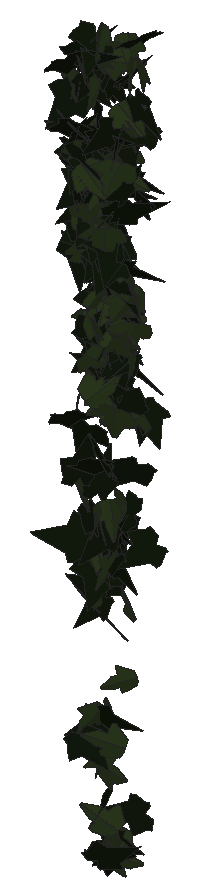
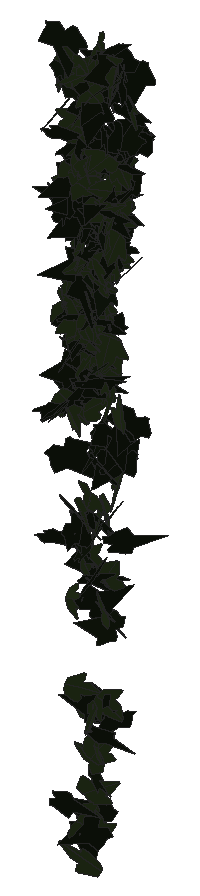
# SketchUp Ruby script. Lengths in millimetres.
U = 1.mm
M = Sketchup.active_model
def pt(a) = Geom::Point3d.new(a.map { |v| v * U })
def face(e, loops, mat)
  f = e.add_face(loops[0].map { |a| pt(a) })
  loops[1..].each { |l| e.add_face(l.map { |a| pt(a) }).erase! }
  f.material = f.back_material = mat if mat
  f
end
# faces: each face lists its corners as indices into pts; further lists are holes
def faces(e, pts, list, mat = nil) = list.each { |f| face(e, (f[0].is_a?(Array) ? f : [f]).map { |l| l.map { |i| pts[i] } }, mat) }
# xy, xz, yz: faces in a plane at the given z, y or x. An outline is a flat list of corners, or four numbers for a rectangle; further outlines are holes
def ring(l) = l.size == 4 ? [[l[0], l[1]], [l[2], l[1]], [l[2], l[3]], [l[0], l[3]]] : l.each_slice(2).to_a
def flat(e, list, mat, &to3) = list.each { |f| face(e, (f[0].is_a?(Array) ? f : [f]).map { |l| ring(l).map { |u, v| to3.(u, v) } }, mat) }
def xy(e, z, list, mat = nil) = flat(e, list, mat) { |x, y| [x, y, z] }
def xz(e, y, list, mat = nil) = flat(e, list, mat) { |x, z| [x, y, z] }
def yz(e, x, list, mat = nil) = flat(e, list, mat) { |y, z| [x, y, z] }
def lines(e, pts, list) = list.each { |a, b| e.add_line(pt(pts[a]), pt(pts[b])) }
# prism: a flat outline (further loops are holes) pulled along v
def prism(e, loops, v, mat = nil)
  f = face(e, loops, mat); d = Geom::Vector3d.new(v.map { |x| x * U })
  f.pushpull(f.normal.samedirection?(d) ? d.length : -d.length)
end
def box(e, o, s, mat = nil) = prism(e, [[o, [o[0] + s[0], o[1], o[2]], [o[0] + s[0], o[1] + s[1], o[2]], [o[0], o[1] + s[1], o[2]]]], [0, 0, s[2]], mat)
def at(x, y, z, deg = 0) = Geom::Transformation.translation(pt([x, y, z])) * Geom::Transformation.rotation(ORIGIN, Z_AXIS, deg.degrees)
def axes(o, x, y, z) = Geom::Transformation.new([*x, 0, *y, 0, *z, 0, *pt(o).to_a, 1])
def part(name) = M.definitions.add(name)
# library, detail: a bought-in or finely detailed component or shape, given as its bounding box
def library(name, o, s) = part(name).tap { |d| box(d.entities, o, s) }
def detail(e, o, s) = box(e.add_group.entities, o, s)
def put(e, d, t, mat = nil) = e.add_instance(d, t).tap { |i| i.material = mat if mat }
def group(e, t, mat = nil) = e.add_group.tap { |g| g.transformation = t; g.material = mat if mat }.entities
root = M.entities
M.materials.add("efeu1").color = [18, 25, 13]
M.materials.add("efeu2").color = [43, 57, 29]
c1 = part("ivyleaf_10")
p = [[0,12.8,-0.8],[-1.5,51.3,-10.9],[-4.9,51,-11.6],[-13.6,26.5,-7.3],[-13.2,15.9,-4.6],[-21.1,19.3,-7.2],
  [-29.5,16.3,-8.3],[-29.2,8.3,-6.2],[-19.7,-9.8,0.5],[-7.6,-13,4],[1,-12.2,5.8],[-0.4,51.1,-11.1],
  [-1.5,51.1,-10.9],[1,-12.4,5.9],[16.9,-12.4,3.5],[35.1,9.1,-5.1],[35,12.9,-6.1],[20.5,16.4,-4.9],
  [15.8,15,-3.8],[15.3,27.6,-7.1],[12.8,31.3,-7.8]]
faces(c1.entities,p,[[0,1,2,3,4,5,6,7,8,9,10],[11,12,0,13,14,15,16,17,18,19,20]],"efeu2")
c2 = part("ivyleaf_9")
p = [[39.1,54.8,31.7],[34.5,51.8,30.2],[-5.3,25.2,17.3],[-17.9,28.3,20.9],[-21.6,21.7,17],[-20.2,4.3,5.3],
  [-22.9,-0.3,2.5],[-17.1,-4,-0.6],[-2,-2.1,-1.2],[-0.7,-15.4,-10.1],[16.6,-22.3,-16.7],[21.1,-15.1,-12.5],
  [32.7,-10.7,-11],[46.1,-1.8,-6.6],[30.8,11.2,3.8]]
faces(c2.entities,p,[[0,1,2,3,4,5,6,7,8,9,10,11,12,13,14]],"efeu1")
put(root,c1,axes([728.7,970.5,1065.7],[-0.31968,0.54228,0.46518],[-0.27067,0.40923,-0.60202],[-0.82856,-0.34291,0.01719]))
put(root,c1,axes([728.9,938,1548.4],[0.79353,-0.55992,-0.23318],[-0.20813,0.15921,-0.85819],[0.71009,0.67238,0.00903]))
put(root,c2,axes([744.1,944,797.2],[-0.53582,-0.01102,0.83666],[-0.94755,-0.34614,-0.41227],[0.37974,-0.87925,0.15182]))
put(root,c1,axes([732.2,963.1,1598.2],[-0.22672,0.60569,0.53252],[-0.43925,0.42669,-0.61097],[-0.88044,-0.36884,0.16768]))
put(root,c2,axes([735.1,935.6,1529.2],[-1.1057,-0.08978,-0.12887],[0.15446,0.02895,-0.9106],[0.11339,-0.91497,-0.01617]))
put(root,c2,axes([724.6,923.5,1004.9],[0.63977,0.58671,-0.02513],[-0.02053,-0.01866,-0.78691],[-0.71615,0.52467,0.00011]))
put(root,c2,axes([732.4,915.9,1591.8],[0.30865,0.90116,-0.0483],[-0.04144,-0.04062,-0.93575],[-1.10022,0.25434,0.0217]))
put(root,c1,axes([720.3,963.6,1016.9],[0.04399,-0.52462,-0.62607],[0.22907,-0.60457,0.51742],[-0.96983,-0.1666,0.09382]))
put(root,c2,axes([718.1,957.9,1264],[0.11253,-0.89011,0.23083],[0.03395,-0.22918,-0.89487],[1.12135,0.09626,0.00393]))
put(root,c1,axes([729.6,962.7,1321.3],[-1.0216,0.33801,-0.11026],[0.12135,-0.04813,-0.90299],[-0.41643,-0.84323,0.00734]))
put(root,c2,axes([722.7,916,1483.5],[1.01081,0.36897,0.02611],[0.02527,0.01767,-0.90694],[-0.45056,0.82875,0.00771]))
put(root,c1,axes([736.4,946.6,1439.5],[-0.19519,-0.77396,0.24193],[-0.04266,-0.23978,-0.7902],[0.98836,-0.1632,0.01367]))
put(root,c2,axes([714.1,932.2,1488.8],[1.27087,-0.47636,-0.12581],[-0.17731,0.08601,-0.8201],[0.92078,0.67404,0.01573]))
put(root,c2,axes([728,924.5,1416.1],[1.04439,-0.15122,-0.43957],[-0.52601,0.08602,-0.86927],[0.21198,0.95846,0.00866]))
put(root,c1,axes([735.4,974.2,1149.6],[-1.01552,-0.2349,-0.07855],[0.08948,0.02929,-0.86487],[0.28863,-0.83558,-0.00823]))
put(root,c2,axes([720.3,956.9,1586.4],[0.01993,-0.07031,-0.84134],[1.0146,-0.14369,0.02816],[-0.17752,-0.82914,0.06646]))
put(root,c2,axes([740.7,951,1375.9],[-0.43673,-0.57022,0.55203],[-0.28276,-0.50408,-0.67098],[0.92606,-0.42283,0.05546]))
put(root,c2,axes([749.2,915.8,1376.6],[0.11456,-0.17142,0.87532],[-0.27883,0.84614,0.19023],[-1.05184,-0.24298,0.0449]))
put(root,c1,axes([736.1,942,1590.3],[-0.4044,0.76317,-0.05677],[0.0276,-0.05207,-0.83204],[-0.93323,-0.33224,-0.00001]))
put(root,c2,axes([754.8,978.2,489.9],[-0.85155,-0.01688,0.31629],[-0.38578,-0.00719,-0.6982],[0.02237,-0.76628,-0.00042]))
put(root,c2,axes([750.7,996.2,1089.6],[-1.07564,-0.43403,0.27698],[-0.36936,-0.20137,-0.71155],[0.90763,-0.59631,0.03868]))
put(root,c2,axes([741.2,920.1,1468.8],[-0.29186,0.57821,-0.62484],[-0.36893,0.54899,0.62381],[0.97088,0.38243,0.04921]))
put(root,c2,axes([748.4,970.9,1359.5],[-0.96537,-0.35342,0.00301],[-0.00304,-0.00181,-0.86663],[0.43118,-0.79129,0.00064]))
put(root,c1,axes([725.8,964.5,1281.9],[0.38067,-0.41931,0.67242],[0.79596,-0.27426,-0.47377],[0.54875,0.68869,0.22074]))
put(root,c1,axes([754.7,978.9,1369],[0.21611,0.36079,0.69796],[-0.64076,-0.47775,0.38026],[0.7129,-0.53877,0.1302]))
put(root,c1,axes([737.9,955,1358.3],[-0.3759,0.74007,-0.17715],[0.09011,-0.16113,-0.80163],[-0.92401,-0.31679,-0.00611]))
put(root,c2,axes([748.9,966.6,1240.7],[0.11528,0.71858,0.40246],[-0.09366,0.41102,-0.71584],[-1.00042,0.04433,0.11339]))
put(root,c1,axes([747.4,964.5,746.2],[0.99954,0.18705,0.36196],[-0.43037,-0.08108,0.84037],[0.24872,-0.89201,-0.00048]))
put(root,c2,axes([749.7,944.8,985.6],[0.50808,0.32888,-0.61181],[-0.56271,-0.40244,-0.5303],[-0.63362,0.62112,-0.01964]))
put(root,c1,axes([737.9,957,1399.3],[0.08746,-0.3433,0.75552],[0.0799,0.75831,0.33836],[-1.00927,0.03028,0.09226]))
put(root,c2,axes([719,981.6,678.8],[0.84735,-0.57903,0.296],[0.33986,-0.23607,-0.73041],[1.19007,0.4797,-0.00216]))
put(root,c1,axes([739.7,972.3,688.8],[0.6757,-0.69026,0.08885],[-0.02864,0.09496,0.88405],[-0.84858,-0.55284,0.04092]))
put(root,c2,axes([741,955.1,1596],[0.34088,0.27983,0.73362],[0.35379,0.68685,-0.37244],[-0.89019,0.38014,0.1329]))
put(root,c1,axes([766.2,932.9,1342.2],[0.18372,0.16574,0.93824],[-1.16191,-0.00062,0.15297],[0.03281,-0.95025,0.16355]))
put(root,c2,axes([745.7,949,1432.1],[-0.80815,-0.5785,-0.1295],[0.21134,-0.00317,-0.8719],[0.69168,-0.67495,0.11509]))
put(root,c1,axes([747.5,947.2,1332.4],[-0.00219,-0.64385,-0.59161],[0.03588,0.59123,-0.64353],[1.06614,-0.02122,0.02044]))
put(root,c2,axes([759.1,979.6,700.9],[0.02789,0.00023,0.88107],[-1.02426,-0.26734,0.02185],[0.32605,-0.83984,-0.00672]))
put(root,c1,axes([733.4,939.4,1373.5],[0.38445,0.26551,0.76924],[0.43253,0.69771,-0.38606],[-0.89363,0.45193,0.14408]))
put(root,c1,axes([749.3,969.5,1218.6],[0.65089,-0.67388,-0.24012],[-0.17006,0.19588,-0.85943],[0.85604,0.55129,0.01185]))
put(root,c2,axes([730.3,978.2,1124.4],[0.48188,-0.71948,-0.02565],[-0.01142,0.02508,-0.76273],[1.37014,0.25325,0.00266]))
put(root,c1,axes([749.3,950,1284.2],[-0.53162,-0.80714,-0.07981],[0.05954,0.06434,-0.91717],[0.98772,-0.43831,0.01234]))
put(root,c1,axes([739.8,960.9,1376.5],[-0.29579,-0.355,-0.68162],[0.49552,0.54758,-0.42966],[0.79597,-0.47281,0.01418]))
put(root,c1,axes([738.1,982.9,1095],[0.67678,-0.4199,0.3753],[0.40876,-0.17736,-0.69367],[0.55225,0.64585,0.0535]))
put(root,c1,axes([747.9,964.9,1282.9],[-0.53394,-0.62456,-0.21132],[0.1501,0.17183,-0.76263],[0.79026,-0.45462,0.00207]))
put(root,c1,axes([751.2,959,1602.6],[-0.10808,-0.71936,0.36185],[-0.04308,-0.36021,-0.72475],[0.98144,-0.09503,0.00804]))
put(root,c2,axes([756.1,951,1355.4],[-0.04711,-0.00353,-0.81943],[-0.03144,-0.81993,0.00475],[-0.99922,0.02597,0.03848]))
put(root,c1,axes([752.4,924.5,896],[-0.63028,0.70695,0.40574],[-0.27479,0.33785,-0.87545],[-0.95571,-0.56336,-0.01586]))
put(root,c1,axes([755.7,980.4,1278.1],[0.66944,-0.41215,-0.40656],[-0.39844,0.24214,-0.68626],[0.58317,0.63856,-0.00218]))
put(root,c2,axes([759.1,968.5,700.4],[-1.01613,0.18831,-0.16249],[0.19034,-0.04672,-0.85384],[-0.23632,-0.84731,0.01097]))
put(root,c2,axes([748.7,962.7,1292.7],[0.71025,0.48394,-0.23634],[-0.21943,-0.15335,-0.75704],[-0.61933,0.60932,-0.00282]))
put(root,c2,axes([738.1,981.8,1579.3],[-0.07761,-0.76036,0.31035],[0.01778,-0.31114,-0.76108],[1.56292,-0.03422,0.02407]))
put(root,c2,axes([740.2,974.8,1477.1],[-0.05471,0.17328,0.80831],[0.13193,-0.80131,0.17778],[0.99987,0.11521,0.02077]))
put(root,c2,axes([751.8,980.2,1181.8],[-0.83416,-0.45971,-0.23375],[0.23675,0.13031,-0.82391],[0.58294,-0.71074,0.00013]))
put(root,c2,axes([745.4,955.6,1300],[-0.46633,-0.75949,-0.28995],[0.19729,0.24297,-0.8496],[0.97199,-0.41369,0.03334]))
put(root,c2,axes([743.2,955.7,1440.5],[0.65086,-0.5158,-0.46393],[-0.3545,0.3653,-0.74028],[0.76855,0.60531,0.05143]))
put(root,c1,axes([750,970.9,1153.6],[0.91405,0.41322,-0.10648],[-0.12741,-0.03105,-0.85531],[-0.50477,0.75612,0.02307]))
put(root,c1,axes([747.9,970.4,1353.3],[-0.28588,0.61191,-0.44511],[0.13833,-0.43231,-0.654],[-0.91272,-0.25718,0.0403]))
put(root,c2,axes([758.4,956.5,1330.1],[-0.57134,0.47847,-0.45991],[0.37688,-0.34103,-0.66935],[-0.71661,-0.56083,0.01465]))
put(root,c2,axes([770.4,980.1,1066.4],[-0.16868,0.03219,0.81843],[-0.99276,-0.09986,-0.13354],[0.11372,-0.824,0.04815]))
put(root,c1,axes([739.9,973.8,1459.1],[0.65674,0.36013,0.5195],[0.51178,0.30691,-0.64744],[-0.57689,0.68225,0.01703]))
put(root,c2,axes([748.4,944.1,1559.1],[0.15361,-0.45757,-0.69364],[-0.26089,0.66008,-0.47425],[0.97963,0.24754,-0.01753]))
put(root,c2,axes([752.9,921.5,917.5],[-0.38926,-0.44734,0.78963],[0.71884,0.5345,0.54089],[-0.84211,0.66304,0.09671]))
put(root,c2,axes([736.3,926.8,1449.6],[0.68597,-0.69001,0.09687],[0.20913,0.01633,-0.87863],[0.82394,0.57032,0.14236]))
put(root,c2,axes([753.6,966.8,1404.1],[0.71699,0.53097,-0.10963],[-0.10768,-0.06583,-0.79197],[-0.65263,0.5942,0.01022]))
put(root,c1,axes([756.8,955.4,1593.5],[-0.93039,0.3137,-0.01831],[0.01853,-0.01121,-0.8246],[-0.38292,-0.76275,0.00459]))
put(root,c1,axes([757.4,986.7,1570.1],[0.35449,0.57132,-0.45747],[-0.26457,-0.40289,-0.64091],[-0.85283,0.36247,0.00867]))
put(root,c1,axes([772,979.7,1164.6],[-0.55609,0.0973,-0.58477],[-0.7097,0.06857,0.46485],[0.13921,0.73825,0.03389]))
put(root,c2,axes([755.4,970.5,748.8],[-0.69747,-0.68993,-0.10118],[0.18061,0.00777,-0.88944],[0.83133,-0.58053,0.10834]))
put(root,c2,axes([746.8,950.8,845.8],[0.58534,-0.68551,-0.32904],[-0.22178,0.27438,-0.8367],[0.90078,0.51301,0.00782]))
put(root,c1,axes([760.1,978.9,1191.5],[-0.51731,-0.68987,-0.02072],[0.02621,0.01112,-0.80967],[0.84161,-0.42438,0.01248]))
put(root,c2,axes([764.1,985.1,736.4],[-0.10856,-0.76389,0.342],[0.10014,0.3343,0.76805],[-1.01616,0.11455,0.03916]))
put(root,c2,axes([758.8,974.3,1541.6],[0.63355,0.56766,-0.23417],[-0.18038,-0.18207,-0.76925],[-0.72712,0.53978,-0.01321]))
put(root,c2,axes([737.7,933.7,1589.9],[0.31223,-0.16925,0.78761],[0.96582,-0.10019,-0.27877],[0.18199,0.82206,0.12818]))
put(root,c1,axes([764.8,947.8,526.5],[-0.17719,-0.64406,0.54774],[-0.13696,-0.53615,-0.6602],[1.02235,-0.18346,0.00649]))
put(root,c1,axes([750.2,984.1,1252.7],[0.88773,-0.10436,0.28946],[0.35323,-0.01936,-0.73481],[0.12707,0.78287,0.02042]))
put(root,c2,axes([755.7,954.2,1623.4],[-0.30481,-0.80875,0.07936],[-0.03159,-0.07506,-0.84646],[0.99091,-0.25117,-0.00258]))
put(root,c1,axes([760.9,940.2,1273.6],[-0.80114,-0.51773,-0.14253],[0.13996,0.0847,-0.83621],[0.64001,-0.6666,0.00445]))
put(root,c2,axes([761.5,965.9,1557.3],[0.27093,0.70084,0.35668],[0.1331,0.33959,-0.73519],[-0.95011,0.24742,-0.00129]))
put(root,c1,axes([762.6,938.2,1164.9],[-0.7686,0.48567,0.12202],[-0.12181,0.07034,-0.79546],[-0.59867,-0.63784,0.00519]))
put(root,c2,axes([752.4,944.1,1338.4],[0.08853,-0.04731,0.88135],[0.75363,0.63436,-0.0168],[-0.76911,0.61614,0.08498]))
put(root,c1,axes([763,965.7,1197.4],[0.05348,-0.8983,0.03926],[0.00479,-0.03912,-0.89937],[1.09697,0.04396,0.00201]))
put(root,c1,axes([768.7,960.5,443.7],[-0.5866,-0.3359,-0.51431],[-0.44453,-0.36987,0.58221],[-0.60335,0.59908,0.07108]))
put(root,c2,axes([755.5,917.1,936.3],[0.78919,0.68241,0.17418],[0.13913,0.13188,-0.94025],[-0.84789,0.65681,0.00783]))
put(root,c1,axes([779.5,969.4,1243.8],[0.22117,0.10389,-0.81011],[-0.99641,0.02684,-0.17933],[0.00454,0.82971,0.10723]))
put(root,c2,axes([766.2,969.4,1233.8],[0.28761,0.80529,-0.13647],[-0.06236,-0.12721,-0.83898],[-0.99451,0.24086,0.01315]))
put(root,c1,axes([777.3,976.2,1156.6],[-0.62875,0.00072,0.61171],[-0.72547,-0.1882,-0.50077],[0.17504,-0.77741,0.12179]))
put(root,c1,axes([757,939.3,1106.6],[-0.36967,-0.41844,-0.62456],[0.43305,0.51396,-0.51655],[0.8085,-0.46662,-0.00889]))
put(root,c2,axes([771.6,954.4,1112.9],[-0.92622,0.38194,-0.05315],[-0.06231,0.01674,0.84982],[0.46632,0.76087,0.00798]))
put(root,c1,axes([771.4,987.6,1409.9],[0.43417,0.38665,-0.56675],[-0.57194,-0.32911,-0.51891],[-0.61113,0.5827,0.08299]))
put(root,c1,axes([767.8,963.7,1604.7],[-0.7145,-0.5761,-0.00496],[-0.0002,0.00724,-0.8215],[0.70287,-0.58563,-0.00528]))
put(root,c1,axes([761.9,936.8,1168.2],[-0.05352,0.71046,0.37985],[-0.02109,0.37949,-0.7118],[-0.98265,-0.04684,-0.00541]))
put(root,c2,axes([756.1,922.8,494.1],[0.13735,-0.5372,-0.63452],[-0.05981,0.63491,-0.54623],[1.01253,0.11038,0.05381]))
put(root,c1,axes([761.4,976.4,1191.5],[0.73236,-0.55914,0.08912],[-0.05521,0.08209,0.81984],[-0.68855,-0.6013,0.02905]))
put(root,c2,axes([769.1,942.3,1351.8],[-0.85046,-0.50232,-0.09959],[0.10218,0.05412,-0.85921],[0.61634,-0.70209,0.00502]))
put(root,c1,axes([763.6,973,519.6],[-0.59279,0.67819,-0.15707],[0.10013,-0.1344,-0.83421],[-0.84337,-0.49265,0.01136]))
put(root,c2,axes([760,938.1,1144],[-0.31705,-0.14346,0.74979],[0.82589,0.32277,0.29639],[-0.43046,0.72494,0.01642]))
put(root,c2,axes([753.7,934,1333],[-0.18965,-0.29097,-0.85133],[0.46693,0.76049,-0.32981],[0.99335,-0.41302,-0.00751]))
put(root,c2,axes([746.4,956.5,1452.3],[0.70518,0.2456,-0.55657],[0.57026,0.31206,0.62315],[0.47501,-0.73925,0.07815]))
put(root,c1,axes([772.1,936.4,850.8],[0.50668,-0.80896,-0.29533],[-0.14226,0.27204,-0.90913],[1.04097,0.43093,0.0195]))
put(root,c1,axes([766,983.9,1449.4],[0.3106,0.74075,-0.09449],[-0.05342,-0.08485,-0.78316],[-0.90947,0.25796,0.01373]))
put(root,c2,axes([770.8,990.8,790.7],[0.377,-0.76459,0.02987],[0.02011,0.03885,0.82413],[-0.93329,-0.30802,0.02982]))
put(root,c2,axes([753.2,983.6,1199.4],[0.55901,-0.59403,0.26107],[0.21542,-0.19339,-0.74993],[0.76174,0.49062,0.02049]))
put(root,c1,axes([749.5,923.3,1335.4],[-0.00282,-0.11604,0.88659],[1.01567,0.32318,0.04447],[-0.39798,0.82559,0.1072]))
put(root,c1,axes([768.2,955.4,1632.8],[-0.07049,0.64432,-0.51881],[-0.04069,-0.52147,-0.6439],[-1.0084,-0.024,0.06225]))
put(root,c1,axes([763.6,960.3,454.3],[0.24093,-0.34368,0.67317],[0.45059,-0.56316,-0.39587],[0.80452,0.41834,0.02012]))
put(root,c1,axes([769,957.2,1195.1],[0.91355,0.31888,-0.08648],[-0.09787,-0.03234,-0.81388],[-0.39102,0.75309,0.00167]))
put(root,c1,axes([771.6,948.4,832.2],[-0.54683,0.79806,0.12168],[-0.07813,0.10359,-0.9153],[-0.98178,-0.45274,0.00507]))
put(root,c1,axes([780.1,965.2,1107.3],[-0.85953,0.05519,0.25441],[-0.3116,-0.00448,-0.70632],[-0.06146,-0.74905,0.02297]))
put(root,c2,axes([771.7,971.7,1436],[-0.75582,-0.11518,0.52343],[0.63971,0.03526,0.62838],[-0.13527,0.81028,0.04706]))
put(root,c2,axes([770.7,947.9,1329.5],[-0.69893,-0.58997,-0.24336],[0.28567,0.1099,-0.81767],[0.72429,-0.61266,0.08767]))
put(root,c2,axes([767.5,952.7,1296.9],[0.67554,-0.34271,-0.54],[-0.45423,0.40804,-0.64074],[0.63444,0.65705,0.11625]))
put(root,c1,axes([774.5,963.7,1020.9],[-0.15477,0.14223,0.83008],[0.08165,-0.83509,0.15331],[1.02421,0.08806,0.11321]))
put(root,c1,axes([771.1,968.8,1094.1],[-0.36519,0.72176,-0.12043],[0.06021,-0.1099,-0.78136],[-0.89069,-0.30336,-0.00344]))
put(root,c1,axes([776.7,927.8,1556.2],[0.66331,-0.70143,-0.14586],[-0.11485,0.11158,-0.88745],[0.86648,0.55175,-0.00597]))
put(root,c2,axes([767.8,970.6,1554.2],[0.52184,-0.52925,-0.44356],[-0.34005,0.34504,-0.68049],[0.77079,0.51054,0.00008]))
put(root,c1,axes([784.7,993.8,565.4],[-0.13688,-0.17915,0.69474],[-0.40315,-0.61125,-0.21099],[0.77694,-0.34874,0.01292]))
put(root,c2,axes([779.1,930.5,899.4],[-0.90698,0.51685,0.11306],[0.10605,-0.07302,0.90538],[0.6367,0.74842,0.01026]))
put(root,c1,axes([773.9,985.1,1092.1],[-0.15436,0.438,0.68865],[0.24202,-0.65947,0.45589],[0.96582,0.23526,-0.00418]))
put(root,c1,axes([777.6,941.6,1353.6],[-0.03773,-0.93867,0.12798],[0.07826,-0.12983,-0.93673],[1.15312,-0.0219,0.06776]))
put(root,c2,axes([775.1,989.4,1191.6],[-0.70286,-0.6875,0.06625],[-0.04456,-0.06262,-0.78036],[1.31376,-0.36994,0.00897]))
put(root,c2,axes([788.1,942.3,1342.9],[-0.47497,0.83839,-0.18068],[0.09532,-0.16292,-0.92437],[-1.04197,-0.39708,-0.0022]))
put(root,c2,axes([786.3,947,832.2],[-1.11227,0.06496,-0.21931],[0.26314,-0.05574,-0.91317],[-0.09286,-0.93604,0.03916]))
put(root,c1,axes([786.7,975.2,859.9],[0.40142,-0.39576,-0.57264],[-0.45806,0.43245,-0.51461],[0.7151,0.49917,-0.00818]))
put(root,c1,axes([767.9,917.8,1421.7],[0.43116,0.72649,0.45874],[0.27102,0.4019,-0.80762],[-1.01259,0.41691,-0.02083]))
put(root,c1,axes([778.5,965.7,767.7],[0.09718,-0.64529,0.60282],[0.12108,-0.5949,-0.64992],[1.07051,0.12586,0.01879]))
put(root,c1,axes([779.8,952.7,1428.1],[0.45231,-0.76465,0.08712],[0.03934,-0.08118,-0.84977],[0.93809,0.37209,-0.00637]))
put(root,c2,axes([793.5,963.5,785.5],[-0.85438,0.57203,-0.08712],[0.08357,-0.05385,-0.90424],[-0.70096,-0.70365,-0.00163]))
put(root,c2,axes([783.8,947.5,1301.9],[-1.02944,-0.27352,-0.27388],[0.34848,0.0033,-0.8833],[0.31869,-0.88713,0.08116]))
put(root,c1,axes([784.2,961.3,1133.1],[0.63895,0.73762,0.06695],[-0.0953,-0.05073,0.81006],[1.40639,-0.33856,0.02448]))
put(root,c1,axes([781.3,987.5,1451.4],[0.10611,-0.7589,0.20736],[0.07088,-0.20186,-0.76313],[0.95717,0.09908,0.03352]))
put(root,c1,axes([784.9,967.8,1178.3],[-0.97958,0.09467,0.08482],[-0.10313,0.00741,-0.80849],[-0.11581,-0.80737,0.00253]))
put(root,c2,axes([767.7,953.7,1226.6],[0.1327,-0.2713,0.72355],[0.29193,-0.68294,-0.29205],[0.89641,0.26257,-0.012]))
put(root,c1,axes([754.8,986.1,271.7],[0.36387,-0.08958,-0.71251],[1.20839,-0.3234,0.21103],[-0.63855,-0.66305,-0.00667]))
put(root,c1,axes([768.3,982.5,1437.6],[0.2481,-0.18768,0.75877],[0.72375,-0.47345,-0.2761],[0.62092,0.62685,0.01865]))
put(root,c1,axes([789.3,983.6,1433.8],[-0.88798,-0.25848,0.20137],[-0.22752,-0.07654,-0.77233],[0.32868,-0.75131,0.0094]))
put(root,c2,axes([778.2,927.1,968],[0.88527,-0.24194,-0.53895],[-0.58661,0.25408,-0.76144],[0.41873,0.86744,0.07271]))
put(root,c2,axes([771.7,953.5,314.7],[0.0446,0.07425,-0.7763],[0.17855,0.7627,0.07984],[0.93451,-0.14926,0.02179]))
put(root,c1,axes([775.4,948.9,1046.9],[0.96,0.34669,0.13669],[0.1501,0.05977,-0.85986],[-0.42916,0.79643,0.00502]))
put(root,c2,axes([779.9,986.5,1124.6],[-0.33731,-0.6071,0.41467],[0.05937,-0.45716,-0.63686],[0.89498,-0.19848,0.19853]))
put(root,c1,axes([797.1,936.2,357.2],[0.51631,0.31993,0.69004],[-0.68201,-0.40463,0.53045],[0.62922,-0.70109,0.00874]))
put(root,c2,axes([785.5,958,1479.9],[-0.04449,-0.17743,-0.81499],[0.384,-0.75838,0.15102],[-0.94234,-0.30066,0.10001]))
put(root,c2,axes([788.2,942.9,402.3],[-0.61897,0.32333,-0.48682],[0.47551,-0.29315,-0.6009],[-0.53125,-0.6391,0.02935]))
put(root,c1,axes([773.1,924.4,1055.4],[0.49238,0.32833,-0.75922],[0.67414,0.52161,0.51931],[0.75095,-0.68354,0.03161]))
put(root,c2,axes([767.9,973.7,1370.3],[0.69789,0.07636,0.53214],[0.64376,0.06884,-0.57712],[-0.12542,0.77825,-0.00116]))
put(root,c1,axes([784,964.7,1348.7],[-0.51544,0.7387,-0.06593],[0.03843,-0.05793,-0.85099],[-0.90398,-0.42366,0.00141]))
put(root,c2,axes([779.4,981.4,1085.5],[-0.56307,-0.26694,-0.56654],[0.73683,-0.0035,-0.49037],[0.20216,-0.73073,0.20931]))
put(root,c2,axes([779.6,975.3,1061],[0.3453,-0.61832,-0.45557],[-0.20676,0.42327,-0.67977],[0.91389,0.32938,0.01834]))
put(root,c1,axes([775.3,956.3,1268.8],[-0.4855,-0.24697,-0.71748],[0.79075,0.31063,-0.46642],[0.48136,-0.75938,0.04255]))
put(root,c1,axes([785.9,938.6,295.9],[-0.81568,-0.38271,0.12977],[0.14694,0.05075,0.77022],[-0.47061,0.67917,0.01557]))
put(root,c1,axes([768.4,957.3,432.2],[0.00673,-0.02259,-0.88683],[0.9276,-0.45677,0.01637],[-0.55758,-0.76017,0.01652]))
put(root,c2,axes([770.1,973.2,822],[0.53263,-0.05962,-0.62087],[0.75663,-0.03908,0.43986],[-0.0809,-0.758,0.02616]))
put(root,c1,axes([790.4,970.4,324.4],[0.22219,0.50974,-0.49504],[-0.25213,-0.45095,-0.54037],[-0.82941,0.27364,0.03165]))
put(root,c2,axes([794.8,946.8,300.3],[0.17898,0.71595,-0.25118],[-0.07386,-0.24397,-0.73076],[-0.92271,0.15841,0.00977]))
put(root,c1,axes([788,980.2,1166.6],[-0.81031,-0.56052,-0.10699],[0.25765,-0.08893,-0.84514],[0.64675,-0.66685,0.20264]))
put(root,c2,axes([768.8,951.9,516.9],[0.5355,-0.14346,0.62728],[0.7232,-0.20524,-0.46173],[0.3054,0.73757,-0.00648]))
put(root,c2,axes([808.7,972.2,850.7],[-0.72082,0.48466,0.36369],[-0.34269,0.23102,-0.76418],[-0.65502,-0.6542,-0.00043]))
put(root,c2,axes([786.6,951,1271.8],[-0.51296,-0.76182,0.23058],[0.14768,-0.31894,-0.83304],[0.95977,-0.35809,0.25142]))
put(root,c1,axes([779.8,968.2,1584],[-0.11833,-0.26119,-0.78817],[0.69376,0.55733,-0.25467],[0.73813,-0.56569,0.11301]))
put(root,c1,axes([792.5,987.2,1020.1],[0.26545,-0.69196,0.11409],[0.0669,-0.10928,-0.70577],[1.33305,0.14327,0.0127]))
put(root,c2,axes([783.9,981,1313.8],[-0.03692,-0.18239,0.77363],[0.02581,-0.7741,-0.18168],[0.96937,0.01366,0.0343]))
put(root,c1,axes([795.9,925.6,1325.9],[-0.89934,-0.56369,0.0175],[-0.01331,-0.01455,-0.92797],[0.6879,-0.73723,0.00493]))
put(root,c1,axes([794.2,933.5,324.1],[-0.00279,0.33527,0.71812],[-0.27753,0.68763,-0.32175],[-0.9262,-0.20705,0.09425]))
put(root,c2,axes([775.9,968.8,767.9],[-0.03503,-0.03299,-0.75949],[0.90188,0.17603,-0.03559],[0.21628,-0.73937,0.02541]))
put(root,c1,axes([796,961.7,1299],[-0.76896,0.60536,0.23266],[-0.21973,0.14828,-0.87375],[-0.76008,-0.6553,0.01722]))
put(root,c2,axes([793.4,963.7,1166.2],[0.65917,0.57065,-0.23637],[-0.21098,-0.16172,-0.78574],[-0.72342,0.56714,0.01377]))
put(root,c1,axes([806.9,969.8,694.2],[-0.36393,0.4073,-0.62117],[-0.51657,0.55876,0.44993],[1.31593,0.33198,0.00483]))
put(root,c2,axes([794.1,981.9,828.9],[-0.26337,0.33588,-0.72797],[0.47404,-0.61561,-0.39926],[-0.85555,-0.44449,0.00288]))
put(root,c2,axes([786.4,961.4,1434],[0.04969,0.36594,0.81738],[-0.14157,-0.80917,0.36805],[1.08337,-0.12252,0.0106]))
put(root,c2,axes([768.5,957.1,1253.7],[1.21088,0.15608,0.45386],[0.83009,0.12651,-0.65492],[-0.38123,0.77122,0.01558]))
put(root,c2,axes([789.1,968.9,1138],[0.52436,-0.39761,-0.54607],[-0.41673,0.43044,-0.58228],[0.71096,0.54556,0.06143]))
put(root,c1,axes([790.1,967.7,1434.9],[-0.07766,-0.21168,-0.86217],[0.03934,-0.86436,0.20984],[-1.08237,-0.01623,0.06949]))
put(root,c1,axes([789.8,974.4,1480.1],[-0.82203,0.37104,-0.24239],[0.26668,-0.10549,-0.7691],[-0.47036,-0.70826,-0.01244]))
put(root,c2,axes([806,976.9,1569.5],[-0.57957,0.62159,-0.18102],[0.0552,-0.1921,-0.77838],[-0.78791,-0.47068,0.07862]))
put(root,c1,axes([812.1,931.3,494.4],[0.18423,0.12074,0.8499],[-0.84579,-0.49174,0.19304],[0.61761,-0.70945,0.01084]))
put(root,c2,axes([788.9,967.2,1334.8],[0.48001,0.43574,0.57124],[0.41764,0.45891,-0.58584],[-0.77063,0.52012,0.03832]))
put(root,c1,axes([785.6,947.8,864.8],[0.90363,-0.23373,0.42112],[0.49737,-0.10708,-0.77647],[0.31287,0.84527,0.01808]))
put(root,c2,axes([816.4,986.3,360.7],[-0.2975,-0.21141,-0.71782],[-0.70584,-0.42556,0.32187],[-0.57901,0.6274,-0.02356]))
put(root,c2,axes([796.9,946.9,1306.8],[-0.53225,-0.81677,-0.07874],[0.03962,0.07192,-0.92597],[1.00029,-0.43744,-0.00522]))
put(root,c2,axes([792.8,974,1464.8],[-0.11912,-0.74613,-0.30074],[0.04535,0.29843,-0.75249],[0.98039,-0.10446,-0.00174]))
put(root,c2,axes([810.5,962.9,1119.4],[-1.0374,-0.00663,-0.06762],[0.08244,0.00571,-0.85034],[0.00862,-0.85299,-0.00517]))
put(root,c2,axes([782.9,969.9,1224.9],[0.39505,-0.80205,0.25688],[0.34205,-0.15685,-0.84316],[0.96885,0.38241,0.19293]))
put(root,c2,axes([818.1,954,1033.8],[0.19445,-0.00668,0.8756],[-0.94156,0.41934,0.14369],[-0.50462,-0.785,0.0693]))
put(root,c1,axes([808.7,933.4,1034.4],[-1.05999,-0.19339,0.14525],[-0.1753,-0.02296,-0.89006],[0.23735,-0.8806,-0.00869]))
put(root,c1,axes([792.9,980.8,1614.8],[0.92321,-0.04398,0.3091],[0.378,0.00602,-0.75768],[0.04689,0.8174,0.02221]))
put(root,c1,axes([788.7,955.2,1157.4],[-0.41429,0.10618,-0.76231],[0.87967,-0.24756,-0.35568],[-0.32845,-0.79696,0.00892]))
put(root,c2,axes([790.2,968.2,1403.1],[0.91976,0.15262,0.31025],[0.36989,0.06595,-0.76919],[-0.20277,0.81258,0.00416]))
put(root,c1,axes([794,968.2,1506.6],[0.6008,0.4161,0.51638],[0.46411,0.34959,-0.64449],[-0.66271,0.62205,0.01679]))
put(root,c1,axes([805.6,984.2,1204.6],[0.91749,-0.43582,0.00601],[0.01821,0.01376,-0.86898],[0.53144,0.75194,0.01939]))
put(root,c2,axes([820.1,932.1,1111.7],[-0.23771,0.94153,0.12857],[-0.08792,0.11622,-0.96034],[-1.15598,-0.20245,0.0466]))
put(root,c1,axes([814.5,952.1,1211.5],[-0.47957,-0.64238,0.30695],[-0.07432,-0.31265,-0.68636],[1.35294,-0.24488,0.0711]))
put(root,c2,axes([821.7,968.5,1585.5],[-0.61685,0.68441,-0.28331],[0.02175,-0.33167,-0.83306],[-0.90343,-0.47529,0.17338]))
put(root,c1,axes([791.8,961.7,1406.8],[-0.38221,-0.15336,-0.74743],[0.92455,0.03143,-0.3241],[0.10826,-0.80983,0.12897]))
put(root,c1,axes([826.9,962.6,1020.3],[-0.62427,0.00828,0.71],[-0.83606,-0.23482,-0.49115],[0.22673,-0.84308,0.14377]))
put(root,c1,axes([816.4,930.3,1436.9],[-0.79283,-0.57022,0.32563],[-0.17094,-0.32717,-0.85254],[0.78266,-0.64908,0.14365]))
put(root,c2,axes([792.3,918.2,306],[0.08622,-0.09791,0.79975],[0.98106,0.0587,-0.06388],[-0.06138,0.80072,0.10247]))
put(root,c2,axes([821.7,963.7,939],[0.00403,0.35405,-0.78387],[-0.30947,-0.74861,-0.33919],[-1.00267,0.23248,0.10154]))
put(root,c2,axes([822.4,988.6,1484.3],[-1.00627,-0.21666,0.16799],[-0.17829,-0.10316,-0.85057],[0.28299,-0.8354,0.06146]))
put(root,c1,axes([810.5,966.6,1227.2],[-0.65649,0.68938,0.05134],[-0.02115,0.05158,-0.87434],[-0.84311,-0.53808,-0.01804]))
put(root,c1,axes([813,944.2,1152.9],[-0.38693,-0.75146,-0.30111],[0.12665,0.28298,-0.81553],[0.97949,-0.33344,-0.0135]))
put(root,c2,axes([794.5,980.6,1087.8],[0.78237,-0.34646,0.28615],[0.31085,-0.13038,-0.72886],[0.45156,0.69002,0.00596]))
put(root,c2,axes([802.6,994.9,1026.7],[0.12864,-0.7065,0.26288],[0.06748,-0.25747,-0.71415],[0.91718,0.11803,0.01567]))
put(root,c2,axes([830.7,942.2,1411.9],[-0.82526,0.66652,0.01684],[-0.01004,0.01564,-0.94963],[-0.81335,-0.67648,-0.00536]))
put(root,c2,axes([801,992.5,1352.2],[0.07165,-0.15285,0.76619],[0.47531,-0.66027,-0.16158],[0.8262,0.39311,0.02651]))
put(root,c2,axes([824.8,961.6,1637.5],[0.17958,0.89947,-0.04674],[-0.17952,-0.02271,-0.90041],[-1.08407,0.15276,0.14137]))
put(root,c1,axes([808.4,968.9,1584.9],[0.37386,-0.58251,0.55429],[0.52189,-0.38417,-0.64023],[0.83064,0.50355,0.15277]))
put(root,c1,axes([821,971.7,1592],[-0.82503,0.58131,0.08761],[-0.13962,0.0008,-0.88872],[-0.70348,-0.68191,0.07364]))
put(root,c1,axes([826.3,954.1,1169.3],[-0.70763,-0.65861,0.2129],[-0.18704,-0.14862,-0.87745],[0.82346,-0.59972,-0.01636]))
put(root,c2,axes([815.8,993.5,1021.1],[-0.1504,-0.7873,0.23501],[0.00597,-0.23834,-0.79589],[1.00237,-0.11671,0.04]))
put(root,c2,axes([832.7,990.3,802.2],[-0.86368,-0.31325,0.23577],[-0.24375,-0.13049,-0.77327],[0.41155,-0.73466,0.03682]))
put(root,c1,axes([833.6,938.9,1134.7],[0.28741,-0.29083,-0.85323],[-0.48108,0.75978,-0.36786],[0.98894,0.45413,0.06902]))
put(root,c2,axes([802.9,942.2,1351.5],[0.29446,0.05272,0.79774],[1.33331,0.38255,-0.16115],[-0.7331,0.71692,0.02733]))
put(root,c2,axes([813.3,976.5,1527.6],[0.56768,-0.625,-0.33915],[-0.20765,0.29563,-0.77833],[0.84231,0.4941,0.03669]))
put(root,c2,axes([813.9,987.2,1025.8],[-0.19054,-0.69718,-0.30488],[0.08679,0.30146,-0.70433],[1.4456,-0.10999,0.0021]))
